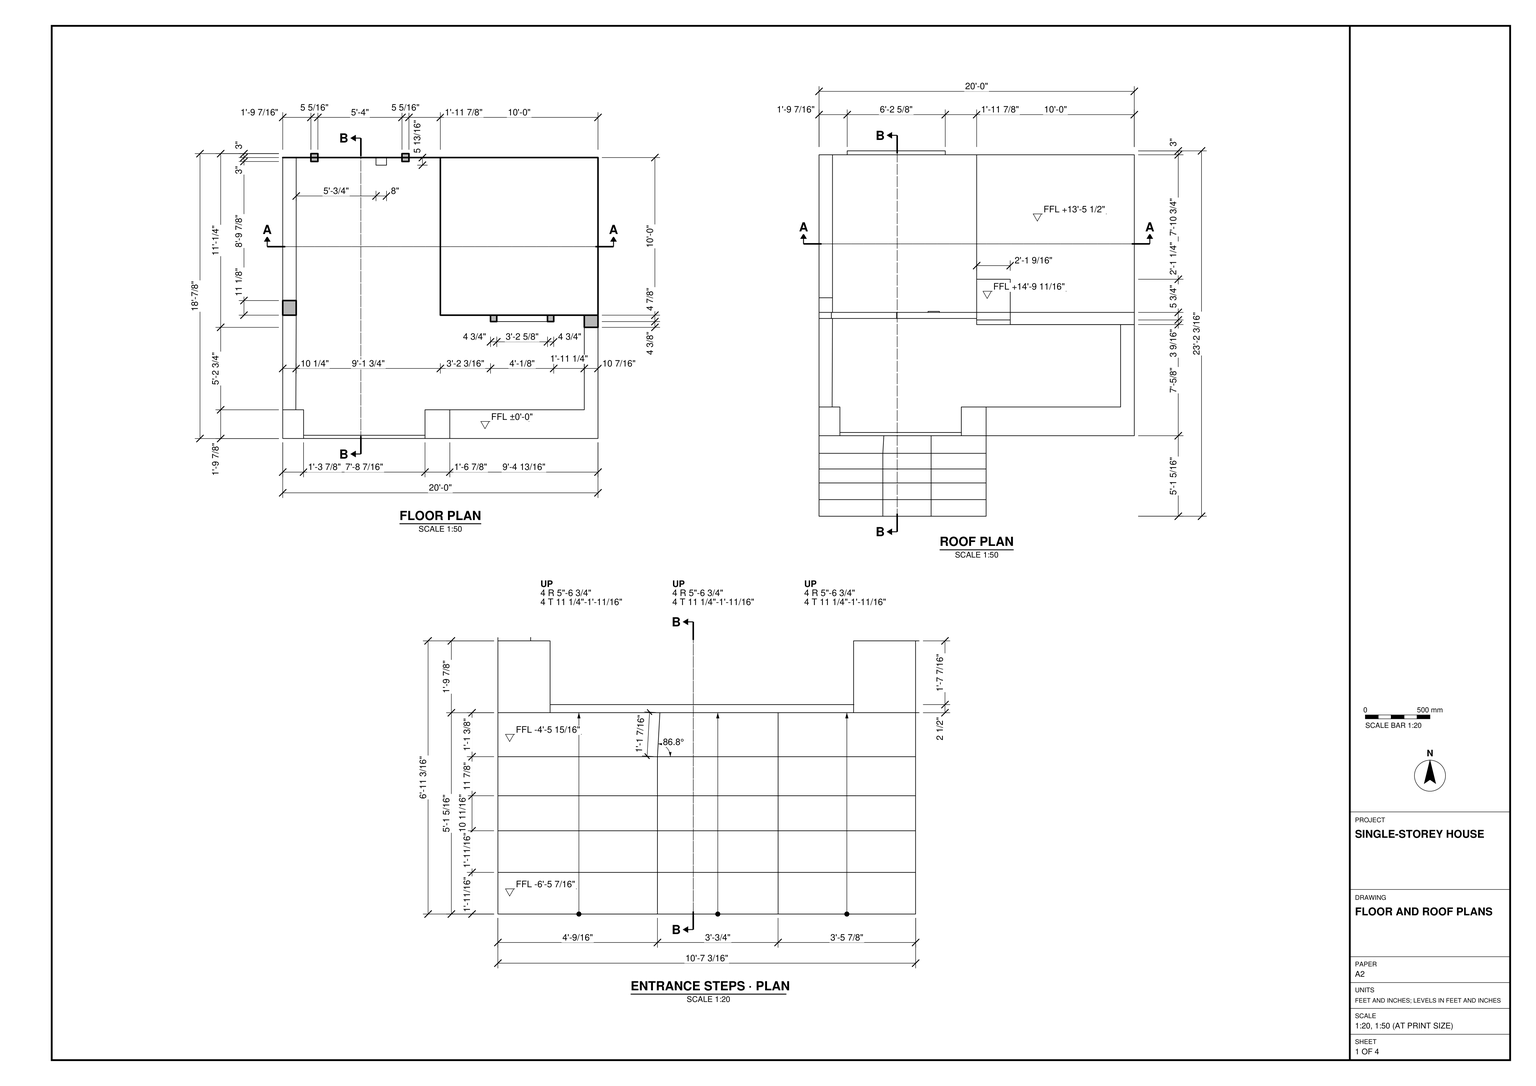
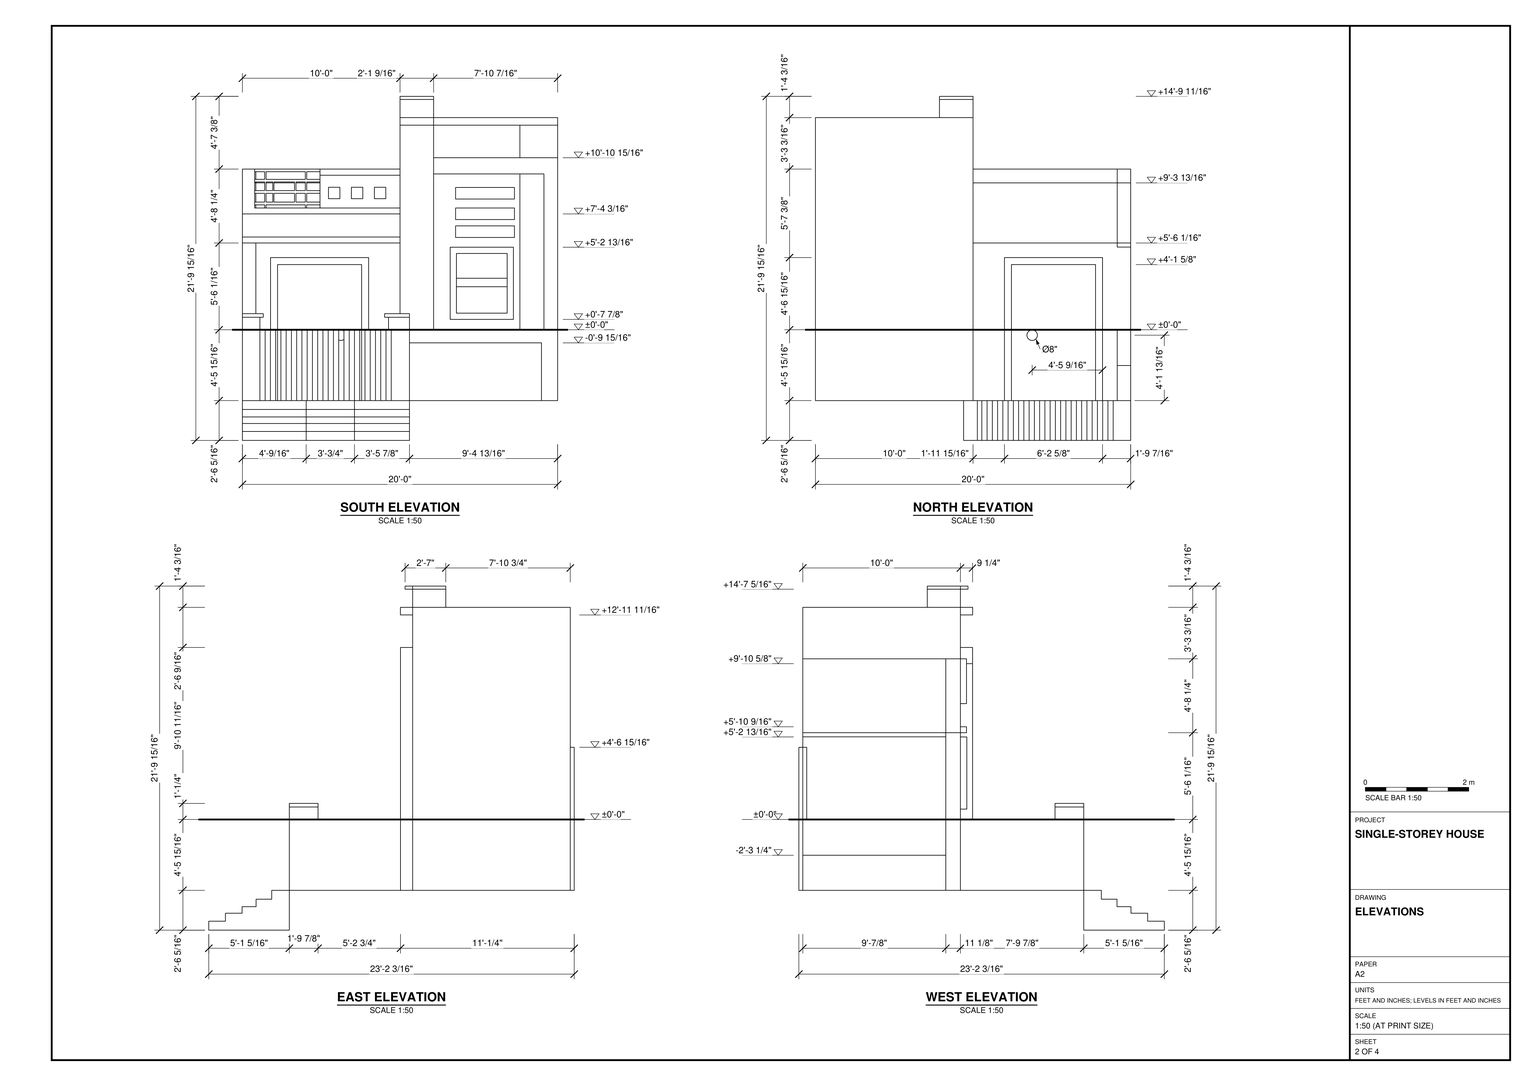
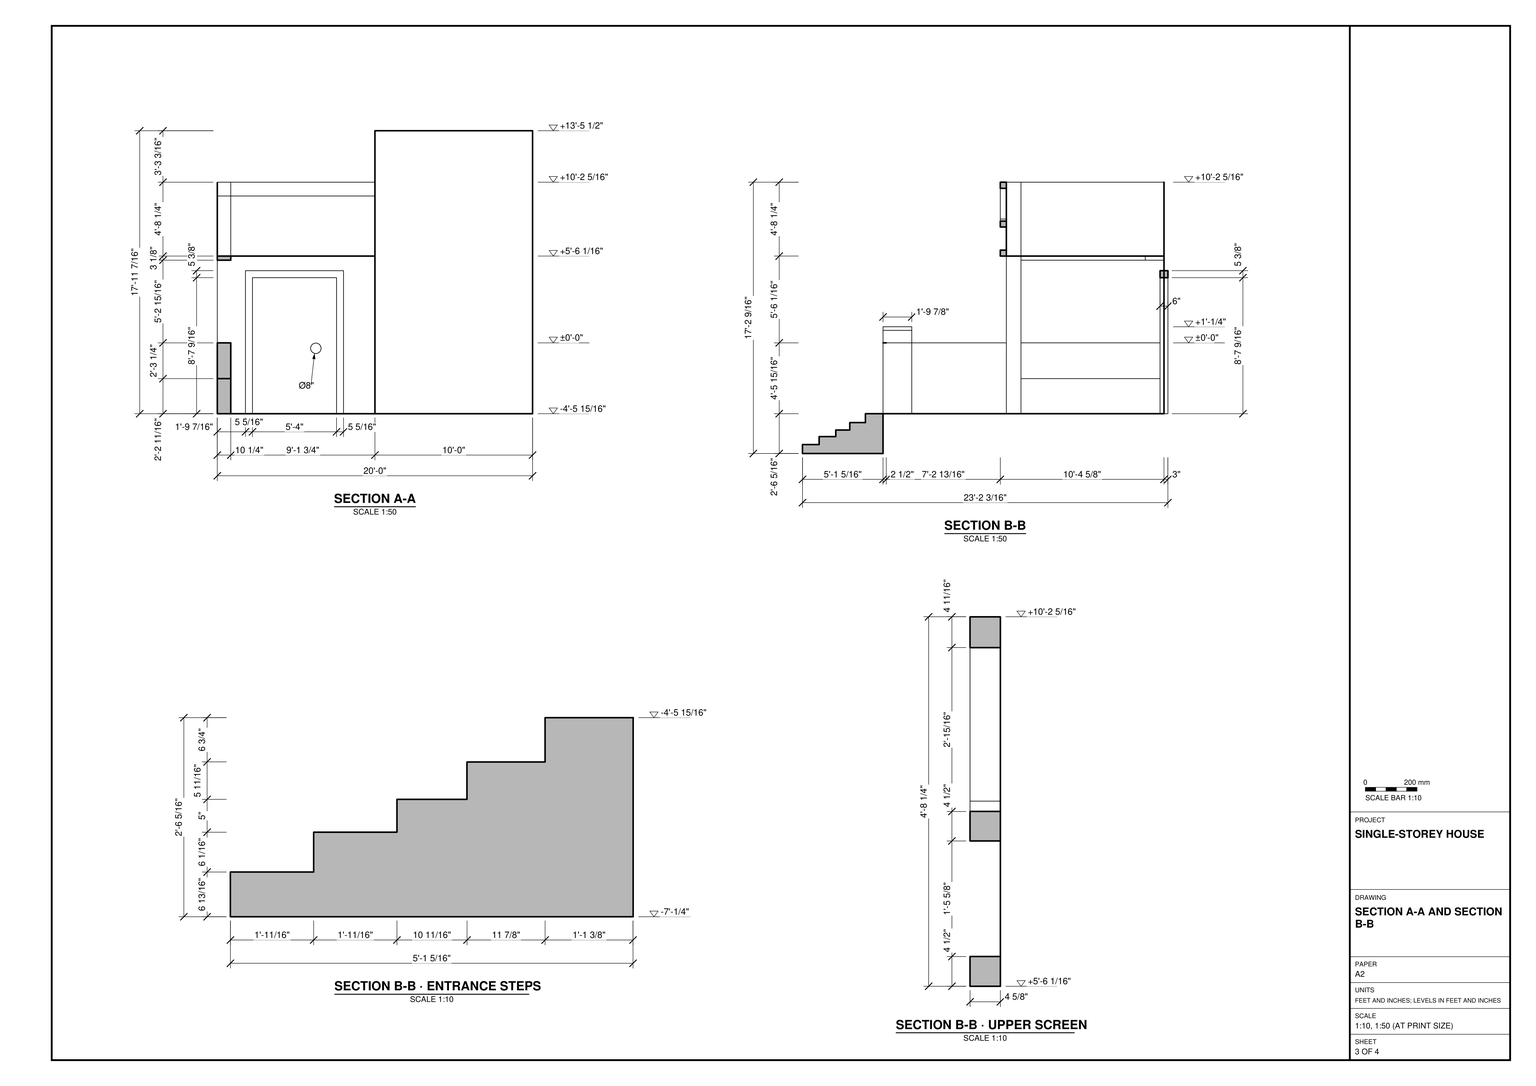
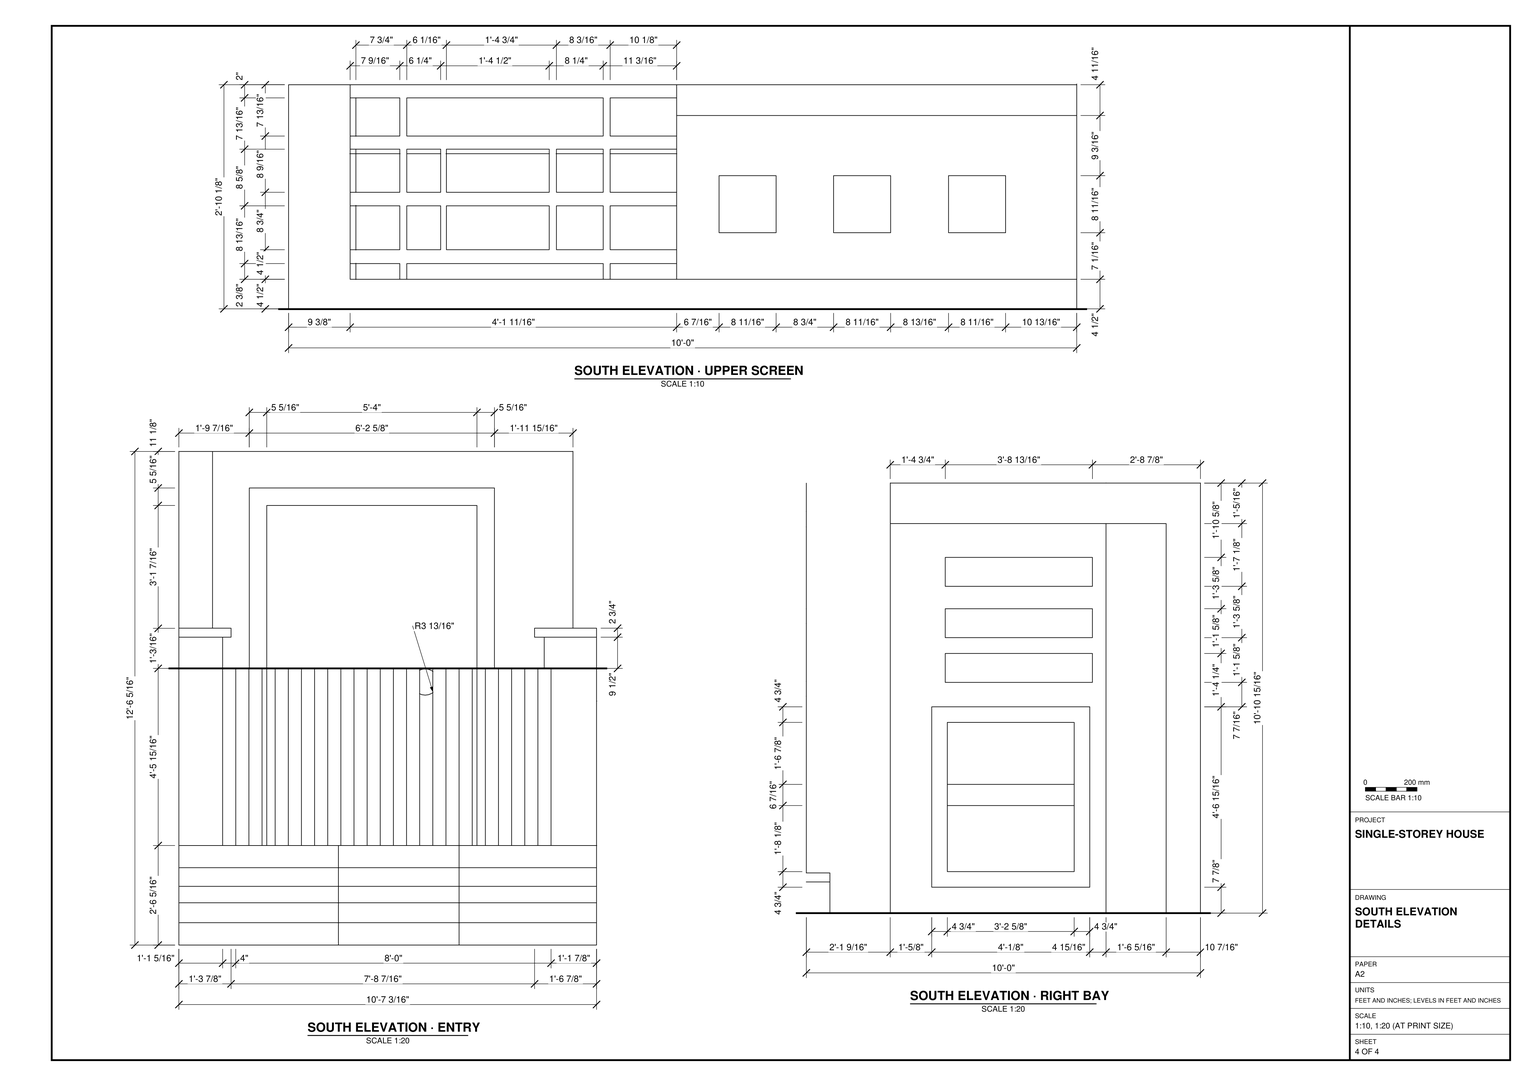
Build the single-storey house in SketchUp from task_files/diagram_01.pdf. Work in feet and inches. Set the ground-floor datum at ±0'-0". The overall model is 20'-0" wide, 23'-2 3/16" deep including the projecting entrance steps, and 21'-9 15/16" high from the bottom of the steps to the highest cap.

Use the floor and roof plans to lay out the walls, their thicknesses and returns, the slabs and the offset roof edges. On the south elevation, distinguish the lower screened bay on the left from the taller bay on the right. Model the framed openings, the horizontal divisions above the right-hand window and the narrow capped projection that rises above the roof. Use the sections to establish the depths of the roof edges and upper screen.

Follow the enlarged entrance plan for the width and tread divisions of the steps, and section B-B for their profile. Align the steps with the vertically divided entrance screen and its capped end posts. Keep walls, slabs and roof elements in separate groups or components. Treat each furniture or joinery piece shown as a separate group or component and use components for repeated parts. Decor and loose items shown may be represented by any suitable library component. Save one SketchUp model as output_files/single_storey_house_with_a_screened_entrance.skp.

# SketchUp Ruby script. Lengths in inches.
U = 1.inch
M = Sketchup.active_model
def pt(a) = Geom::Point3d.new(a.map { |v| v * U })
def face(e, loops, mat)
  f = e.add_face(loops[0].map { |a| pt(a) })
  loops[1..].each { |l| e.add_face(l.map { |a| pt(a) }).erase! }
  f.material = f.back_material = mat if mat
  f
end
# faces: each face lists its corners as indices into pts; further lists are holes
def faces(e, pts, list, mat = nil) = list.each { |f| face(e, (f[0].is_a?(Array) ? f : [f]).map { |l| l.map { |i| pts[i] } }, mat) }
# xy, xz, yz: faces in a plane at the given z, y or x. An outline is a flat list of corners, or four numbers for a rectangle; further outlines are holes
def ring(l) = l.size == 4 ? [[l[0], l[1]], [l[2], l[1]], [l[2], l[3]], [l[0], l[3]]] : l.each_slice(2).to_a
def flat(e, list, mat, &to3) = list.each { |f| face(e, (f[0].is_a?(Array) ? f : [f]).map { |l| ring(l).map { |u, v| to3.(u, v) } }, mat) }
def xy(e, z, list, mat = nil) = flat(e, list, mat) { |x, y| [x, y, z] }
def xz(e, y, list, mat = nil) = flat(e, list, mat) { |x, z| [x, y, z] }
def yz(e, x, list, mat = nil) = flat(e, list, mat) { |y, z| [x, y, z] }
def lines(e, pts, list) = list.each { |a, b| e.add_line(pt(pts[a]), pt(pts[b])) }
# prism: a flat outline (further loops are holes) pulled along v
def prism(e, loops, v, mat = nil)
  f = face(e, loops, mat); d = Geom::Vector3d.new(v.map { |x| x * U })
  f.pushpull(f.normal.samedirection?(d) ? d.length : -d.length)
end
def box(e, o, s, mat = nil) = prism(e, [[o, [o[0] + s[0], o[1], o[2]], [o[0] + s[0], o[1] + s[1], o[2]], [o[0], o[1] + s[1], o[2]]]], [0, 0, s[2]], mat)
def at(x, y, z, deg = 0) = Geom::Transformation.translation(pt([x, y, z])) * Geom::Transformation.rotation(ORIGIN, Z_AXIS, deg.degrees)
def axes(o, x, y, z) = Geom::Transformation.new([*x, 0, *y, 0, *z, 0, *pt(o).to_a, 1])
def part(name) = M.definitions.add(name)
# library, detail: a bought-in or finely detailed component or shape, given as its bounding box
def library(name, o, s) = part(name).tap { |d| box(d.entities, o, s) }
def detail(e, o, s) = box(e.add_group.entities, o, s)
def put(e, d, t, mat = nil) = e.add_instance(d, t).tap { |i| i.material = mat if mat }
def group(e, t, mat = nil) = e.add_group.tap { |g| g.transformation = t; g.material = mat if mat }.entities
root = M.entities
M.materials.add("[0020_Red]").color = [255, 0, 0]
M.materials.add("[0107_MidnightBlue]").color = [25, 25, 112]
M.materials.add("[0110_LightSlateGray]").color = [119, 136, 153]
M.materials.add("[0128_White]").color = [255, 255, 255]
M.materials.add("[0137_Black]").color = [0, 0, 0]
M.materials.add("[Brick Tumbled]").color = [135, 132, 132]
M.materials.add("[Carrera Marble]").color = [207, 207, 207]
M.materials.add("[Color C06]").color = [204, 102, 0]
M.materials.add("[Metal Seamed]").color = [118, 119, 115]
M.materials.add("[Translucent Glass Sky Reflection]").color = [126, 138, 183]
M.materials["[Translucent Glass Sky Reflection]"].alpha = 0.52
M.materials.add("[Wood Cherry Original]").color = [152, 86, 42]
M.materials.add("[Wood Veneer 01]").color = [120, 70, 37]
xy(root,-30.3125,[[0,0,127.18,61.32]])
xy(root,-23.5,[[0,0,48.58,12.68],[85.32,0,127.18,12.68]])
xy(root,-23.5,[[48.58,0,85.32,12.68]],"[0107_MidnightBlue]")
xy(root,-17.4375,[[0,12.68,48.58,25.36],[85.32,12.68,127.18,25.36]])
xy(root,-17.4375,[[48.58,12.68,85.32,25.36]],"[0107_MidnightBlue]")
xy(root,-12.4375,[[0,25.36,48.58,36.02],[85.32,25.36,127.18,36.02]])
xy(root,-12.4375,[[48.58,25.36,85.32,36.02]],"[0107_MidnightBlue]")
xy(root,-6.75,[[0,36.02,48.58,47.91],[85.32,36.02,127.18,47.91]])
xy(root,-6.75,[[48.58,36.02,85.32,47.91]],"[0107_MidnightBlue]")
xy(root,0,[[0,47.91,48.58,47.91,49.32,61.32,0,61.32],[85.32,47.91,127.18,61.32],[0,61.32,0,155.21,229.5625,155.21,229.5625,83.2,111.25,83.2,111.25,61.32],[111.25,61.32,111.25,83.2,229.5625,83.2,229.5625,145.96,240,145.96,240,61.32],[229.5625,145.96,240,155.21],
  [0,155.21,10.25,166.34],[10.25,155.21,10.25,275.21,21.4375,275.21,21.4375,272.21,26.76,272.21,26.76,275.21,90.76,275.21,90.76,272.21,96.09,272.21,96.09,275.21,120,275.21,120,155.21],[120,155.21,240,275.21],[0,166.34,10.25,275.21]])
xy(root,0,[[48.58,47.91,85.32,47.91,85.32,61.32,49.32,61.32]],"[0107_MidnightBlue]")
xy(root,0,[[21.4375,272.21,26.76,275.21],[90.76,272.21,96.09,275.21],[21.4375,275.21,26.76,278.21],[90.76,275.21,96.09,278.21]],"[Color C06]")
xy(root,26.71,[[0,166.34,10.25,275.21]])
xy(root,53.9375,[[0,61.32,13.32,83.2],[111.25,61.32,127.18,83.2],[127.18,61.32,240,61.32,240,145.96,229.5625,145.96,229.5625,83.2,127.18,83.2],[0,83.2,9.97,83.2,10.25,155.21,0,155.21]])
xy(root,53.9375,[[0,166.34,10.25,275.21]],"[0128_White]")
xy(root,53.9375,[[13.32,61.32,111.25,63.78]],"[Metal Seamed]")
xy(root,61.83,[[158.18,150.33,206.31,155.21]])
xy(root,63.4375,[[0,61.32,13.32,83.2],[13.32,61.32,15.88,83.2],[108.31,61.32,111.25,83.2],[111.25,61.32,127.18,83.2]])
xy(root,66.1875,[[0,61.32,15.88,83.2],[108.31,61.32,127.18,83.2]],"[0128_White]")
xy(root,66.58,[[162.93,150.33,201.5625,155.21]])
xy(root,103.55,[[26.76,275.21,90.76,278.21]],"[Color C06]")
xy(root,103.55,[[26.76,272.21,90.76,275.21]],"[Wood Cherry Original]")
xy(root,108.88,[[21.4375,275.21,96.09,278.21]],"[Color C06]")
xy(root,108.88,[[21.4375,272.21,96.09,275.21]],"[Wood Cherry Original]")
xy(root,112.02,[[162.93,150.33,201.5625,155.21]])
xy(root,116.77,[[158.18,150.33,206.31,155.21]])
xy(root,116.875,[[0,166.34,10.25,275.21]])
xy(root,120,[[0,150.58,10.25,155.21],[10.25,150.58,120,155.21],[0,155.21,10.25,166.34],[0,166.34,10.25,275.21]])
xy(root,120,[[10.25,155.21,120,275.21]],"[Wood Veneer 01]")
xy(root,124.53,[[0,150.58,120,155.21]])
xy(root,142.13,[[0,150.58,120,155.21]])
xy(root,146.625,[[9.375,150.58,59.09,155.21],[59.09,150.58,120,155.21]])
xy(root,153.72,[[65.54,153.08,74.23,155.21],[82.98,153.08,91.67,155.21],[100.48,153.08,109.17,155.21],[82.98,155.21,91.67,155.96]])
xy(root,162.41,[[65.54,153.08,74.23,155.21],[82.98,153.08,91.67,155.21],[100.48,153.08,109.17,155.21],[82.98,155.21,91.67,155.96]])
xy(root,171.5625,[[59.09,150.58,120,155.21]])
xy(root,172.57,[[145.5625,145.96,229.5625,155.21]])
xy(root,176.25,[[0,150.58,9.375,155.21],[59.09,150.58,120,155.21]])
xy(root,184.9,[[145.5625,145.96,240,155.21]],"[0128_White]")
xy(root,209.66,[[120,145.9,145.5625,155.21],[145.5625,145.9,240,155.21]],"[0128_White]")
xy(root,215.4375,[[120,145.9,145.5625,155.21],[145.5625,145.9,240,155.21],[120,155.21,145.5625,180.45]])
xy(root,215.4375,[[145.5625,155.21,240,155.21,240,275.21,120,275.21,120,180.45,145.5625,180.45]],"[0128_White]")
xy(root,229.25,[[120,149.46,145.5625,155.21],[120,155.21,145.5625,180.45]])
xy(root,231.625,[[120,149.46,145.5625,155.21],[120,155.21,145.5625,180.45]])
xz(root,0,[[48.58,-30.3125,85.32,-23.5]],"[0107_MidnightBlue]")
xz(root,0,[[0,-30.3125,48.58,-23.5],[85.32,-30.3125,127.18,-23.5]],"[0128_White]")
xz(root,12.68,[[48.58,-23.5,85.32,-17.4375]],"[0107_MidnightBlue]")
xz(root,12.68,[[0,-23.5,48.58,-17.4375],[85.32,-23.5,127.18,-17.4375]],"[0128_White]")
xz(root,25.36,[[48.58,-17.4375,85.32,-12.4375]],"[0107_MidnightBlue]")
xz(root,25.36,[[0,-17.4375,48.58,-12.4375],[85.32,-17.4375,127.18,-12.4375]],"[0128_White]")
xz(root,36.02,[[48.58,-12.4375,85.32,-6.75]],"[0107_MidnightBlue]")
xz(root,36.02,[[0,-12.4375,48.58,-6.75],[85.32,-12.4375,127.18,-6.75]],"[0128_White]")
xz(root,47.91,[[48.58,-6.75,85.32,0]],"[0107_MidnightBlue]")
xz(root,47.91,[[0,-6.75,48.58,0],[85.32,-6.75,127.18,0]],"[0128_White]")
xz(root,61.32,[[0,-30.3125,13.32,0],[13.32,-30.3125,17.32,0],[17.32,-30.3125,21.32,0],[21.32,-30.3125,25.32,0],[25.32,-30.3125,29.32,0],
  [29.32,-30.3125,33.32,0],[33.32,-30.3125,37.32,0],[37.32,-30.3125,41.32,0],[41.32,-30.3125,45.32,0],[45.32,-30.3125,49.32,0],
  [49.32,-30.3125,53.32,0],[53.32,-30.3125,57.32,0],[57.32,-30.3125,61.32,0],[61.32,-30.3125,65.32,0],[65.32,-30.3125,69.32,0],
  [69.32,-30.3125,73.32,0],[73.32,-30.3125,77.32,0],[77.32,-30.3125,81.32,0],[81.32,-30.3125,85.32,0],[85.32,-30.3125,89.32,0],
  [89.32,-30.3125,93.32,0],[93.32,-30.3125,97.32,0],[97.32,-30.3125,101.32,0],[101.32,-30.3125,105.32,0],[105.32,-30.3125,109.32,0],
  [109.32,-30.3125,113.32,0],[113.32,-30.3125,116.74,0],[116.74,-30.3125,127.18,0],[108.31,63.4375,127.18,66.1875]])
xz(root,61.32,[[0,0,13.32,53.9375],[113.32,0,127.18,53.9375],[0,53.9375,13.32,63.4375],[111.25,53.9375,127.18,63.4375]],"[0110_LightSlateGray]")
xz(root,61.32,[[227.68,0,240,0,240,53.9375,127.18,53.9375,127.18,43.98,227.68,43.98],[0,63.4375,15.88,66.1875]],"[0128_White]")
xz(root,61.32,[[127.18,0,227.68,43.98]],"[Brick Tumbled]")
xz(root,61.32,[[13.32,0,17.32,53.9375],[21.32,0,25.32,53.9375],[29.32,0,33.32,53.9375],[37.32,0,41.32,53.9375],[45.32,0,49.32,53.9375],
  [53.32,0,57.32,53.9375],[61.32,0,65.32,53.9375],[69.32,0,73.32,53.9375],[77.32,0,81.32,53.9375],[85.32,0,89.32,53.9375],
  [93.32,0,97.32,53.9375],[101.32,0,105.32,53.9375],[109.32,0,113.32,53.9375]],"[Metal Seamed]")
xz(root,83.2,[[111.25,0,229.5625,53.9375],[0,53.9375,9.97,63.4375],[9.97,53.9375,13.32,63.4375],[111.25,53.9375,127.18,63.4375],[0,63.4375,9.97,66.1875],
  [9.97,63.4375,13.32,66.1875],[13.32,63.4375,15.88,66.1875],[108.31,63.4375,111.25,66.1875],[111.25,63.4375,127.18,66.1875]])
xz(root,145.9,[[120,209.66,145.5625,215.4375],[145.5625,209.66,240,215.4375]],"[0128_White]")
xz(root,145.96,[[229.5625,0,240,53.9375]])
xz(root,145.96,[[229.5625,53.9375,240,53.9375,240,184.9,145.5625,184.9,145.5625,172.57,229.5625,172.57]],"[0128_White]")
xz(root,149.46,[[120,229.25,145.5625,231.625]])
xz(root,150.33,[[[158.18,61.83,206.31,116.77],[162.93,66.58,201.5625,112.02]]],"[0128_White]")
xz(root,150.58,[[0,120,120,124.53],[0,142.13,120,142.13,120,146.625,9.375,146.625,9.375,176.25,0,176.25]])
xz(root,150.58,[[59.09,171.5625,120,176.25]],"[0128_White]")
xz(root,153.08,[[65.54,153.72,74.23,162.41],[82.98,153.72,91.67,162.41],[100.48,153.72,109.17,162.41]],"[0128_White]")
xz(root,155.21,[[0,0,10.25,53.9375],[229.5625,0,229.5625,172.57,145.5625,172.57,145.5625,184.9,240,184.9,240,0],[0,53.9375,10.25,120],[[158.18,61.83,206.31,116.77],[162.93,66.58,201.5625,112.02]],[0,120,120,124.53],
  [0,142.13,0,176.25,9.375,176.25,9.375,146.625,120,146.625,120,142.13],[65.54,153.72,74.23,162.41],[82.98,153.72,91.67,162.41],[100.48,153.72,109.17,162.41],[59.09,171.5625,120,176.25],
  [120,209.66,145.5625,215.4375],[145.5625,209.66,240,215.4375],[120,229.25,145.5625,231.625]])
xz(root,155.21,[[120,0,145.5625,209.66],[120,215.4375,145.5625,229.25]],"[0020_Red]")
xz(root,155.21,[[162.3,124.2,207.11,133.02],[162.3,137.83,207.11,146.64],[162.3,153.45,207.11,162.27]],"[0107_MidnightBlue]")
xz(root,155.21,[[[145.5625,0,211.25,172.57],[158.18,61.83,206.31,116.77],[162.3,153.45,207.11,162.27],[162.3,137.83,207.11,146.64],[162.3,124.2,207.11,133.02]],[[59.09,146.625,120,171.5625],[82.98,153.72,91.67,162.41],[100.48,153.72,109.17,162.41],[65.54,153.72,74.23,162.41]],[145.5625,184.9,211.25,209.66]],"[0110_LightSlateGray]")
xz(root,155.21,[[162.93,86.69,201.5625,93.15]],"[0137_Black]")
xz(root,155.21,[[211.25,0,229.5625,172.57],[0,124.53,120,142.13],[211.25,184.9,240,209.66]],"[Brick Tumbled]")
xz(root,155.21,[[[16.9375,146.625,18,146.625,18,149.02,47.9,149.02,47.9,146.625,48.96,146.625,48.96,149.02,59.09,149.02,59.09,151.13,48.96,151.13,48.96,157.8125,59.09,157.8125,59.09,159.875,48.96,159.875,48.96,166.4375,59.09,166.4375,59.09,168.4375,48.96,168.4375,48.96,174.25,59.09,174.25,59.09,176.25,9.375,176.25,9.375,174.25,16.9375,174.25,16.9375,168.4375,9.375,168.4375,9.375,166.4375,16.9375,166.4375,16.9375,159.875,9.375,159.875,9.375,157.8125,16.9375,157.8125,16.9375,151.13,9.375,151.13,9.375,149.02,16.9375,149.02],[18,168.4375,47.9,174.25],[24.03,151.13,39.6875,157.8125],[24.03,159.875,39.6875,166.4375],[40.78,151.13,47.9,157.8125],[40.78,159.875,47.9,166.4375],[18,151.13,23.16,157.8125],[18,159.875,23.16,166.4375]]],"[Metal Seamed]")
xz(root,155.21,[[162.93,66.58,201.5625,86.69],[162.93,93.15,201.5625,112.02]],"[Translucent Glass Sky Reflection]")
xz(root,155.96,[[82.98,153.72,91.67,162.41]])
xz(root,166.34,[[0,0,10.25,26.71],[0,26.71,10.25,53.9375],[0,53.9375,10.25,116.875],[0,116.875,10.25,120]])
xz(root,180.45,[[120,229.25,145.5625,231.625]])
xz(root,180.45,[[120,215.4375,145.5625,229.25]],"[0020_Red]")
xz(root,269.4,[[75,45.8,76.04,45.93,77,46.33,77.83,46.97,78.47,47.8,78.87,48.76,79,49.8,78.87,50.83,78.47,51.8,77.83,52.625,77,53.26,76.04,53.66,75,53.8,73.97,53.66,73,53.26,72.18,52.625,71.54,51.8,71.14,50.83,71,49.8,71.14,48.76,71.54,47.8,72.18,46.97,73,46.33,73.97,45.93]],"[Metal Seamed]")
xz(root,272.21,[[21.4375,0,26.76,0,26.76,103.55,90.76,103.55,90.76,0,96.09,0,96.09,108.88,21.4375,108.88]],"[Wood Cherry Original]")
xz(root,275.21,[[0,0,10.25,26.71],[120,0,240,215.4375],[0,26.71,10.25,53.9375],[0,116.875,10.25,120],[0,120,10.25,165.75],
  [10.25,120,120,165.75],[0,165.75,10.25,176.25],[10.25,165.75,120,176.25]])
xz(root,275.21,[[10.25,0,10.25,53.9375,0,53.9375,0,116.875,10.25,116.875,10.25,120,120,120,120,0,96.09,0,96.09,108.88,21.4375,108.88,21.4375,0]],"[Carrera Marble]")
xz(root,275.21,[[21.4375,0,21.4375,108.88,96.09,108.88,96.09,0,90.76,0,90.76,103.55,26.76,103.55,26.76,0]],"[Color C06]")
xz(root,275.21,[[[26.76,0,90.76,103.55],[75,45.8,76.04,45.93,77,46.33,77.83,46.97,78.47,47.8,78.87,48.76,79,49.8,78.87,50.83,78.47,51.8,77.83,52.625,77,53.26,76.04,53.66,75,53.8,73.97,53.66,73,53.26,72.18,52.625,71.54,51.8,71.14,50.83,71,49.8,71.14,48.76,71.54,47.8,72.18,46.97,73,46.33,73.97,45.93]],[75,45.8,73.97,45.93,73,46.33,72.18,46.97,71.54,47.8,71.14,48.76,71,49.8,71.14,50.83,71.54,51.8,72.18,52.625,73,53.26,73.97,53.66,75,53.8,76.04,53.66,77,53.26,77.83,52.625,78.47,51.8,78.87,50.83,79,49.8,78.87,48.76,78.47,47.8,77.83,46.97,77,46.33,76.04,45.93]],"[Wood Cherry Original]")
xz(root,278.21,[[21.4375,0,21.4375,108.88,96.09,108.88,96.09,0,90.76,0,90.76,103.55,26.76,103.55,26.76,0]],"[Color C06]")
yz(root,0,[[0,-30.3125,0,-23.5,12.68,-23.5,12.68,-17.4375,25.36,-17.4375,25.36,-12.4375,36.02,-12.4375,36.02,-6.75,47.91,-6.75,47.91,0,61.32,0,61.32,-30.3125],[166.34,116.875,275.21,120],[150.58,120,155.21,124.53],[150.58,142.13,155.21,176.25]])
yz(root,0,[[61.32,0,155.21,53.9375],[155.21,0,166.34,53.9375],[166.34,0,275.21,26.71],[166.34,26.71,275.21,53.9375],[61.32,53.9375,83.2,63.4375],
  [155.21,53.9375,166.34,120],[61.32,63.4375,83.2,66.1875],[155.21,120,166.34,176.25],[166.34,120,275.21,176.25]],"[0128_White]")
yz(root,9.375,[[150.58,146.625,155.21,148.1875],[150.58,148.1875,155.21,176.25]])
yz(root,10.25,[[155.21,0,166.34,120],[166.34,116.875,260.94,120],[260.94,116.875,275.21,120]])
yz(root,10.25,[[166.34,0,275.21,26.71],[166.34,26.71,275.21,53.9375]],"[0128_White]")
yz(root,13.32,[[61.32,53.9375,83.2,63.4375]],"[0110_LightSlateGray]")
yz(root,15.88,[[61.32,63.4375,83.2,66.1875]])
yz(root,21.4375,[[275.21,0,278.21,108.88]],"[Color C06]")
yz(root,21.4375,[[272.21,0,275.21,108.88]],"[Wood Cherry Original]")
yz(root,26.76,[[275.21,0,278.21,103.55]],"[Color C06]")
yz(root,26.76,[[272.21,0,275.21,103.55]],"[Wood Cherry Original]")
yz(root,59.09,[[150.58,171.5625,155.21,176.25]])
yz(root,65.54,[[153.08,153.72,155.21,162.41]])
yz(root,74.23,[[153.08,153.72,155.21,162.41]])
yz(root,82.98,[[153.08,153.72,155.21,162.41],[155.21,153.72,155.96,162.41]])
yz(root,90.76,[[275.21,0,278.21,103.55]],"[Color C06]")
yz(root,90.76,[[272.21,0,275.21,103.55]],"[Wood Cherry Original]")
yz(root,91.67,[[153.08,153.72,155.21,162.41],[155.21,153.72,155.96,162.41]])
yz(root,96.09,[[275.21,0,278.21,108.88]],"[Color C06]")
yz(root,96.09,[[272.21,0,275.21,108.88]],"[Wood Cherry Original]")
yz(root,100.48,[[153.08,153.72,155.21,162.41]])
yz(root,108.31,[[61.32,63.4375,83.2,66.1875]],"[0128_White]")
yz(root,109.17,[[153.08,153.72,155.21,162.41]])
yz(root,111.25,[[61.32,53.9375,83.2,63.4375]],"[0110_LightSlateGray]")
yz(root,120,[[155.21,0,275.21,120],[150.58,120,155.21,124.53],[155.21,120,275.21,165.75],[150.58,142.13,155.21,146.625],[155.21,165.75,275.21,176.25],
  [150.58,171.5625,155.21,176.25],[155.21,176.25,275.21,215.4375],[145.9,209.66,155.21,215.4375],[149.46,229.25,155.21,231.625],[155.21,229.25,180.45,231.625]])
yz(root,120,[[155.21,215.4375,180.45,229.25]],"[0020_Red]")
yz(root,127.18,[[0,-30.3125,61.32,-30.3125,61.32,0,47.91,0,47.91,-6.75,36.02,-6.75,36.02,-12.4375,25.36,-12.4375,25.36,-17.4375,12.68,-17.4375,12.68,-23.5,0,-23.5],[61.32,53.9375,83.2,63.4375],[61.32,63.4375,83.2,66.1875]])
yz(root,145.5625,[[145.96,172.57,155.21,184.9],[145.9,209.66,155.21,215.4375],[149.46,229.25,155.21,231.625],[155.21,229.25,180.45,231.625]])
yz(root,145.5625,[[155.21,215.4375,180.45,229.25]],"[0020_Red]")
yz(root,158.18,[[150.33,61.83,155.21,116.77]])
yz(root,162.93,[[150.33,66.58,155.21,86.69],[150.33,86.69,155.21,93.15],[150.33,93.15,155.21,112.02]])
yz(root,201.5625,[[150.33,66.58,155.21,86.69],[150.33,86.69,155.21,93.15],[150.33,93.15,155.21,112.02]])
yz(root,206.31,[[150.33,61.83,155.21,116.77]])
yz(root,229.5625,[[83.2,0,145.96,53.9375],[145.96,0,155.21,172.57]])
yz(root,240,[[61.32,0,145.96,53.9375],[145.96,0,155.21,184.9]])
yz(root,240,[[155.21,0,275.21,215.4375],[145.9,209.66,155.21,215.4375]],"[0128_White]")
p = [[9.97,83.2,0],[10.25,155.21,0],[10.25,155.21,53.9375],[9.97,83.2,53.9375],[73.97,275.21,45.93],[75,275.21,45.8],
  [75,269.4,45.8],[73.97,269.4,45.93],[76.04,275.21,45.93],[76.04,269.4,45.93],[73,275.21,46.33],[73,269.4,46.33],
  [77,275.21,46.33],[77,269.4,46.33],[72.18,275.21,46.97],[72.18,269.4,46.97],[77.83,275.21,46.97],[77.83,269.4,46.97],
  [71.54,275.21,47.8],[71.54,269.4,47.8],[78.47,275.21,47.8],[78.47,269.4,47.8],[71.14,275.21,48.76],[71.14,269.4,48.76],
  [78.87,275.21,48.76],[78.87,269.4,48.76],[71,275.21,49.8],[71,269.4,49.8],[79,275.21,49.8],[79,269.4,49.8],
  [71.14,275.21,50.83],[71.14,269.4,50.83],[78.87,275.21,50.83],[78.87,269.4,50.83],[71.54,275.21,51.8],[71.54,269.4,51.8],
  [78.47,275.21,51.8],[78.47,269.4,51.8],[72.18,275.21,52.625],[72.18,269.4,52.625],[77.83,275.21,52.625],[77.83,269.4,52.625],
  [73,275.21,53.26],[73,269.4,53.26],[77,275.21,53.26],[77,269.4,53.26],[73.97,275.21,53.66],[73.97,269.4,53.66],
  [76.04,275.21,53.66],[76.04,269.4,53.66],[75,275.21,53.8],[75,269.4,53.8],[10.25,166.34,120],[10.25,166.34,165.75]]
faces(root,p,[[0,1,2,3]])
faces(root,p,[[4,5,6,7],[5,8,9,6],[10,4,7,11],[8,12,13,9],[14,10,11,15],[12,16,17,13],[18,14,15,19],[16,20,21,17],
  [22,18,19,23],[20,24,25,21],[26,22,23,27],[24,28,29,25],[30,26,27,31],[28,32,33,29],[34,30,31,35],[32,36,37,33],
  [38,34,35,39],[36,40,41,37],[42,38,39,43],[40,44,45,41],[46,42,43,47],[44,48,49,45],[50,46,47,51],[48,50,51,49]],"[Metal Seamed]")
lines(root,p,[[52,53]])
